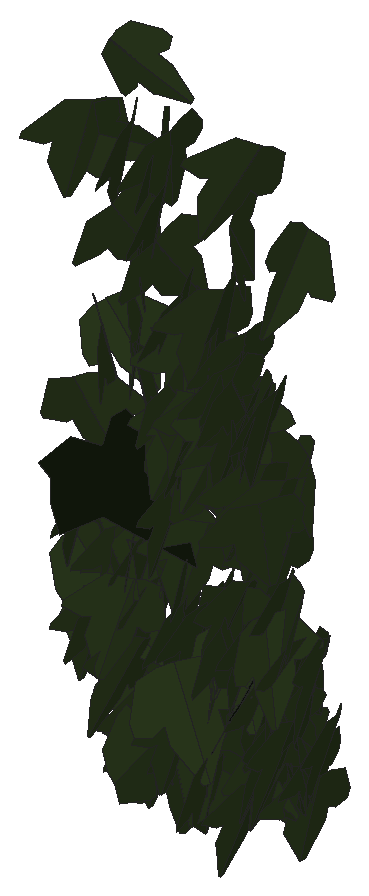
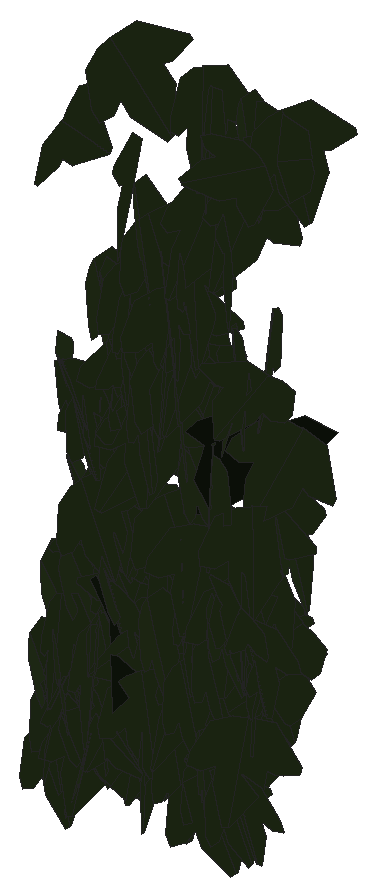
# SketchUp Ruby script. Lengths in inches.
U = 1.inch
M = Sketchup.active_model
def pt(a) = Geom::Point3d.new(a.map { |v| v * U })
def face(e, loops, mat)
  f = e.add_face(loops[0].map { |a| pt(a) })
  loops[1..].each { |l| e.add_face(l.map { |a| pt(a) }).erase! }
  f.material = f.back_material = mat if mat
  f
end
# faces: each face lists its corners as indices into pts; further lists are holes
def faces(e, pts, list, mat = nil) = list.each { |f| face(e, (f[0].is_a?(Array) ? f : [f]).map { |l| l.map { |i| pts[i] } }, mat) }
# xy, xz, yz: faces in a plane at the given z, y or x. An outline is a flat list of corners, or four numbers for a rectangle; further outlines are holes
def ring(l) = l.size == 4 ? [[l[0], l[1]], [l[2], l[1]], [l[2], l[3]], [l[0], l[3]]] : l.each_slice(2).to_a
def flat(e, list, mat, &to3) = list.each { |f| face(e, (f[0].is_a?(Array) ? f : [f]).map { |l| ring(l).map { |u, v| to3.(u, v) } }, mat) }
def xy(e, z, list, mat = nil) = flat(e, list, mat) { |x, y| [x, y, z] }
def xz(e, y, list, mat = nil) = flat(e, list, mat) { |x, z| [x, y, z] }
def yz(e, x, list, mat = nil) = flat(e, list, mat) { |y, z| [x, y, z] }
def lines(e, pts, list) = list.each { |a, b| e.add_line(pt(pts[a]), pt(pts[b])) }
# prism: a flat outline (further loops are holes) pulled along v
def prism(e, loops, v, mat = nil)
  f = face(e, loops, mat); d = Geom::Vector3d.new(v.map { |x| x * U })
  f.pushpull(f.normal.samedirection?(d) ? d.length : -d.length)
end
def box(e, o, s, mat = nil) = prism(e, [[o, [o[0] + s[0], o[1], o[2]], [o[0] + s[0], o[1] + s[1], o[2]], [o[0], o[1] + s[1], o[2]]]], [0, 0, s[2]], mat)
def at(x, y, z, deg = 0) = Geom::Transformation.translation(pt([x, y, z])) * Geom::Transformation.rotation(ORIGIN, Z_AXIS, deg.degrees)
def axes(o, x, y, z) = Geom::Transformation.new([*x, 0, *y, 0, *z, 0, *pt(o).to_a, 1])
def part(name) = M.definitions.add(name)
# library, detail: a bought-in or finely detailed component or shape, given as its bounding box
def library(name, o, s) = part(name).tap { |d| box(d.entities, o, s) }
def detail(e, o, s) = box(e.add_group.entities, o, s)
def put(e, d, t, mat = nil) = e.add_instance(d, t).tap { |i| i.material = mat if mat }
def group(e, t, mat = nil) = e.add_group.tap { |g| g.transformation = t; g.material = mat if mat }.entities
root = M.entities
M.materials.add("efeu1").color = [18, 25, 13]
M.materials.add("efeu2").color = [43, 57, 29]
c1 = part("ivyleaf_10")
p = [[0,0.5,-0.03],[-0.0625,2.02,-0.43],[-0.19,2.01,-0.46],[-0.54,1.05,-0.29],[-0.52,0.625,-0.18],[-0.83,0.76,-0.28],
  [-1.16,0.64,-0.33],[-1.15,0.33,-0.24],[-0.77,-0.39,0.02],[-0.3,-0.51,0.16],[0.04,-0.48,0.23],[-0.02,2.01,-0.4375],
  [-0.06,2.01,-0.43],[0.04,-0.49,0.23],[0.67,-0.49,0.14],[1.38,0.36,-0.2],[1.375,0.51,-0.24],[0.81,0.65,-0.19],
  [0.62,0.59,-0.15],[0.6,1.09,-0.28],[0.5,1.23,-0.31]]
faces(c1.entities,p,[[0,1,2,3,4,5,6,7,8,9,10],[11,12,0,13,14,15,16,17,18,19,20]],"efeu2")
c2 = part("ivyleaf_9")
p = [[1.54,2.16,1.25],[1.36,2.04,1.19],[-0.21,0.99,0.68],[-0.71,1.11,0.82],[-0.85,0.86,0.67],[-0.8,0.17,0.21],
  [-0.9,-0.01,0.1],[-0.67,-0.16,-0.02],[-0.08,-0.08,-0.05],[-0.03,-0.6,-0.4],[0.65,-0.88,-0.66],[0.83,-0.6,-0.49],
  [1.29,-0.42,-0.43],[1.8125,-0.07,-0.26],[1.21,0.44,0.15]]
faces(c2.entities,p,[[0,1,2,3,4,5,6,7,8,9,10,11,12,13,14]],"efeu1")
put(root,c1,axes([511.15,138.33,173.45],[-0.53133,-0.36546,-0.08051],[0.06901,0.04172,-0.64486],[0.3678,-0.53577,0.0047]))
put(root,c1,axes([511.1875,137.57,174.37],[-0.07517,-0.63344,0.13711],[0.02718,-0.14099,-0.63646],[0.64754,-0.06761,0.04263]))
put(root,c1,axes([511.03,137.4,177.95],[-0.62883,-0.1578,-0.2539],[0.25357,0.03165,-0.64769],[0.15833,-0.67742,0.02889]))
put(root,c1,axes([511.2,137.5,174.31],[-0.0367,-0.5542,-0.34902],[0.05334,0.34587,-0.55481],[0.65276,-0.05942,0.02571]))
put(root,c1,axes([511.25,137.1,176.54],[0.20511,-0.67223,-0.01479],[0.00018,0.01552,-0.70281],[0.6724,0.20506,0.0047]))
put(root,c1,axes([510.8,137.61,175.09],[0.46308,0.08973,0.46146],[0.45781,0.13491,-0.45439],[-0.1716,0.6021,0.03304]))
put(root,c1,axes([511.34,137.03,182.93],[-0.29651,-0.63131,0.13286],[-0.02442,-0.13513,-0.69661],[0.64468,-0.29549,0.03472]))
put(root,c1,axes([510.87,138.625,183.2],[-0.29498,-0.01649,-0.51058],[0.5277,-0.06697,-0.28036],[-0.05464,-0.5578,0.04875]))
put(root,c1,axes([510.94,138.64,175.75],[0.4809,-0.09085,0.34008],[0.34546,-0.06796,-0.47263],[0.12251,0.54826,-0.00224]))
put(root,c1,axes([511.21,138.05,175.04],[0.65936,-0.04096,-0.05098],[-0.04671,0.06659,-0.65758],[0.04577,0.65796,0.06338]))
put(root,c1,axes([511.38,137.85,176.66],[-0.52077,-0.41886,0.03252],[-0.00711,-0.043,-0.66769],[0.42006,-0.52001,0.02902]))
put(root,c1,axes([511.26,138.24,172.6],[0.65161,-0.20335,0.02645],[0.02522,-0.00797,-0.68261],[0.20351,0.6521,-0.0001]))
put(root,c1,axes([511.12,137.7,175.75],[-0.52464,0.14683,-0.37282],[0.31847,-0.23272,-0.5147],[-0.27132,-0.55707,0.11676]))
put(root,c1,axes([511.45,137.89,175.45],[-0.20993,-0.6397,-0.03572],[0.00516,0.0359,-0.67324],[0.64068,-0.2099,-0.00628]))
put(root,c1,axes([510.98,137.7,174.26],[0.33472,0.27444,0.5275],[0.38809,0.35781,-0.4324],[-0.45052,0.51212,0.01943]))
put(root,c1,axes([511.49,137.92,175.6],[0.35504,-0.46871,-0.31687],[-0.08504,0.32563,-0.57696],[0.55935,0.34702,0.11341]))
put(root,c1,axes([511.5,138.23,172.43],[-0.02758,-0.61533,0.16209],[0.03251,-0.16339,-0.61474],[0.63549,-0.01834,0.03848]))
put(root,c1,axes([511.57,137.98,175.37],[-0.3656,-0.54994,-0.10257],[0.08431,0.06697,-0.65956],[0.55304,-0.37376,0.03275]))
put(root,c1,axes([511.6,137.75,173.51],[0.00758,-0.57265,0.3385],[0.00865,-0.3384,-0.57269],[0.66516,0.01093,0.00359]))
put(root,c1,axes([511.25,137.83,179.11],[0.42155,0.29513,0.33107],[0.27307,0.19342,-0.50891],[-0.38109,0.46506,0.00156]))
put(root,c1,axes([511.7,138.06,175.33],[0.10458,-0.6555,0.0077],[-0.01596,-0.01034,-0.66356],[0.65535,0.10436,-0.01739]))
put(root,c1,axes([511.7,136.9,179.41],[0.38995,-0.4563,-0.37185],[-0.01203,0.43978,-0.55226],[0.58851,0.31134,0.23511]))
put(root,c1,axes([511.77,137.43,174.71],[-0.35506,-0.50671,0.22798],[0.00311,-0.27236,-0.60051],[0.55563,-0.32228,0.14905]))
put(root,c1,axes([511.26,137.13,182.5625],[0.17142,-0.08418,0.61824],[0.46785,0.44179,-0.05523],[-0.44896,0.42824,0.1785]))
put(root,c1,axes([511.9375,138.21,172.18],[-0.38663,-0.46937,0.22543],[-0.07868,-0.22489,-0.6032],[0.51472,-0.38694,0.07713]))
put(root,c1,axes([511.85,138.16,174.59],[0.04878,-0.6554,-0.01014],[-0.0002,0.01015,-0.65721],[0.65548,0.04877,0.00056]))
put(root,c1,axes([511.93,137.45,179.28],[0.41217,-0.49191,-0.26423],[-0.06963,0.28057,-0.63096],[0.55402,0.40123,0.11728]))
put(root,c1,axes([511.95,138.22,172.9],[0.20759,-0.57519,-0.19],[-0.04277,0.18643,-0.61111],[0.60425,0.2108,0.02202]))
put(root,c1,axes([512.01,137.625,172.52],[-0.0152,-0.64209,-0.11858],[0.01256,0.11831,-0.6422],[0.65283,-0.01723,0.00959]))
put(root,c1,axes([512.06,137.06,182.87],[0.23939,-0.66517,-0.10263],[-0.01169,0.10481,-0.70652],[0.67294,0.23844,0.02423]))
put(root,c1,axes([512.34,137.12,180.95],[-0.21157,0.41784,0.51326],[-0.42359,0.32854,-0.44207],[-0.50853,-0.44751,0.15469]))
put(root,c1,axes([512.04,136.95,181.56],[-0.26905,-0.54368,-0.37865],[0.17077,0.33796,-0.60661],[0.64015,-0.31866,0.00268]))
put(root,c1,axes([512.16,137.83,172.32],[-0.08214,-0.66371,0.02105],[-0.0003,-0.02118,-0.66877],[0.66405,-0.08211,0.00231]))
put(root,c1,axes([512.15,137.7,177.2],[0.49209,-0.44172,-0.14903],[0.05273,0.26804,-0.62036],[0.46319,0.43877,0.22895]))
put(root,c1,axes([512.02,137.51,178.69],[-0.36654,0.44971,-0.37639],[0.21445,-0.31033,-0.57963],[-0.54582,-0.42393,0.02503]))
put(root,c1,axes([512.28,137.85,176.02],[-0.59455,-0.29765,-0.08444],[0.09273,0.00307,-0.66378],[0.29517,-0.60051,0.03846]))
put(root,c1,axes([512.18,136.92,172.2],[0.0671,0.21097,-0.64366],[0.2053,0.61005,0.22136],[0.64549,-0.21596,-0.00349]))
put(root,c2,axes([511.98,136.68,177.61],[-0.05901,-0.38165,-0.68878],[0.1505,0.67252,-0.38553],[0.77293,-0.16009,0.02248]))
put(root,c1,axes([512.55,137.88,173.7],[-0.01342,-0.65638,0.0168],[-0.00529,-0.01669,-0.6565],[0.65658,-0.01355,-0.00495]))
put(root,c1,axes([512.67,137.08,182.85],[0.19003,-0.57376,-0.38438],[-0.05336,0.38528,-0.60148],[0.68855,0.18821,0.05947]))
put(root,c1,axes([512.7,137.92,172.49],[-0.02827,-0.65385,-0.01163],[-0.00667,0.01193,-0.65443],[0.65392,-0.02815,-0.00717]))
put(root,c1,axes([512.79,136.93,182.1],[0.19013,-0.65849,-0.24032],[-0.07022,0.22986,-0.68538],[0.69744,0.20265,-0.00349]))
put(root,c1,axes([512.79,137.64,175.64],[0.2884,-0.57359,-0.24048],[-0.02182,0.25558,-0.63578],[0.62158,0.27511,0.08925]))
put(root,c1,axes([512.81,137.41,174.77],[0.07086,-0.64045,-0.17021],[0.00638,0.17183,-0.6439],[0.66265,0.06683,0.0244]))
put(root,c1,axes([512.85,137.57,173.5],[-0.01933,-0.49141,-0.47177],[0.04592,0.46995,-0.49139],[0.67967,-0.04572,0.01978]))
put(root,c1,axes([512.93,137.1875,180.21],[0.0808,-0.66352,-0.23934],[-0.04887,0.23506,-0.66816],[0.70368,0.09251,-0.01892]))
put(root,c1,axes([512.82,137.01,181.1875],[-0.23526,-0.54082,-0.40317],[0.15837,0.37077,-0.58977],[0.65571,-0.28359,-0.00221]))
put(root,c1,axes([512.93,136.99,183.06],[-0.10108,-0.67884,-0.18934],[0.00661,0.19036,-0.68601],[0.70472,-0.09915,-0.02072]))
put(root,c1,axes([512.91,138.18,174.76],[0.13352,-0.64214,-0.01462],[-0.00702,0.01347,-0.65586],[0.64227,0.13364,-0.00412]))
put(root,c1,axes([512.95,137.34,173.11],[-0.0679,-0.63604,0.13574],[0.00556,-0.13704,-0.63935],[0.65034,-0.06524,0.01964]))
put(root,c1,axes([512.91,137.21,176.95],[0.13014,-0.63696,0.17304],[0.03828,-0.16879,-0.65011],[0.65894,0.13561,0.00359]))
put(root,c1,axes([513.19,137.14,171.78],[0.46474,-0.12951,0.46006],[-0.44306,0.12388,0.48245],[-0.17922,-0.6421,0.00029]))
put(root,c1,axes([512.99,137.03,178.82],[-0.1159,-0.54203,-0.39898],[0.11383,0.38324,-0.55371],[0.66335,-0.16047,0.02531]))
put(root,c1,axes([513.13,137.53,176.13],[-0.33046,-0.55119,0.19166],[-0.04559,-0.19519,-0.63997],[0.58177,-0.32838,0.05871]))
put(root,c1,axes([513.1,137.29,178.36],[-0.18619,-0.6015,0.31164],[0.00284,-0.32389,-0.62344],[0.67743,-0.16396,0.08827]))
put(root,c1,axes([513.21,137.36,179.48],[-0.51677,-0.47524,0.07532],[0.04077,-0.15338,-0.68803],[0.47944,-0.4992,0.13969]))
put(root,c1,axes([513.22,138.05,173.37],[-0.41186,-0.51185,0.09508],[0.02956,-0.14403,-0.64733],[0.51977,-0.3974,0.11216]))
put(root,c1,axes([513.24,137.4,174.94],[0.01032,-0.6808,-0.11343],[-0.01706,0.11316,-0.68071],[0.68997,0.01298,-0.01513]))
put(root,c1,axes([513.27,137.08,178.16],[0.24069,-0.62018,-0.23706],[-0.05204,0.23376,-0.66438],[0.6619,0.24389,0.03397]))
put(root,c1,axes([513.24,137.4375,179.93],[0.51893,-0.45673,-0.11867],[-0.00277,0.17343,-0.67962],[0.47189,0.50328,0.12651]))
put(root,c1,axes([513.29,137.3,178.72],[0.2338,-0.5929,-0.29713],[0.0359,0.32591,-0.62207],[0.66222,0.19166,0.13863]))
put(root,c1,axes([513.4,137.42,178.44],[-0.12113,-0.62782,0.29259],[-0.02907,-0.29216,-0.63893],[0.69204,-0.12216,0.02437]))
put(root,c1,axes([513.4375,137.6,177.77],[-0.58298,-0.36605,-0.00176],[-0.00323,0.00847,-0.68832],[0.36604,-0.58292,-0.00889]))
put(root,c1,axes([513.39,137.69,172.36],[0.17197,-0.5681,-0.25628],[0.00695,0.26759,-0.58851],[0.6232,0.15379,0.07728]))
put(root,c1,axes([513.21,137.05,178.18],[-0.47799,-0.28981,-0.39055],[0.35687,0.16301,-0.55773],[0.33039,-0.59534,0.03741]))
put(root,c1,axes([513.53,137.59,178.02],[0.08114,-0.66509,-0.15393],[-0.02152,0.15245,-0.67002],[0.68234,0.0839,-0.00283]))
put(root,c1,axes([513.68,137.95,171.97],[-0.24863,-0.32018,-0.50653],[-0.32199,-0.39112,0.40527],[-0.50538,0.40671,-0.00902]))
put(root,c1,axes([513.58,137.18,174.44],[0.42995,-0.46886,-0.18478],[-0.03177,0.21719,-0.62502],[0.50296,0.41453,0.11848]))
put(root,c1,axes([513.3,136.78,173.98],[0.58767,0.37901,0.26824],[0.21856,0.15596,-0.69919],[-0.40968,0.62689,0.01177]))
put(root,c1,axes([513.625,136.95,172.61],[0.19809,-0.62649,-0.21894],[0.01193,0.23181,-0.65252],[0.66354,0.18286,0.07709]))
put(root,c1,axes([513.69,137.18,180.45],[-0.20553,-0.66648,0.16178],[-0.01653,-0.16403,-0.69673],[0.68564,-0.20374,0.0317]))
put(root,c1,axes([513.48,137.4,177.46],[-0.3782,-0.44886,-0.43311],[0.29899,0.31407,-0.58657],[0.54742,-0.48164,0.02114]))
put(root,c1,axes([514.14,138.15,172.61],[-0.06744,0.12528,0.62325],[-0.63293,0.04537,-0.07761],[-0.05944,-0.62524,0.11925]))
put(root,c1,axes([513.71,137.34,178.35],[-0.10111,-0.51814,0.45118],[0.09384,-0.46218,-0.50974],[0.68061,-0.01325,0.1373]))
put(root,c1,axes([513.7,137.32,173.88],[-0.01572,-0.03598,-0.69138],[0.13889,0.67733,-0.03841],[0.67824,-0.13954,-0.00815]))
put(root,c1,axes([514.02,138.32,173.98],[-0.45545,0.33583,0.4292],[-0.35538,0.24103,-0.56572],[-0.41316,-0.57754,0.01348]))
put(root,c1,axes([513.81,137.36,178.13],[-0.11679,-0.67361,0.04651],[0.06611,-0.05838,-0.67954],[0.67197,-0.11133,0.07494]))
put(root,c1,axes([513.71,137.69,173.13],[-0.35736,-0.43856,-0.36402],[0.22763,0.28409,-0.56572],[0.52253,-0.42369,-0.00252]))
put(root,c1,axes([514,137.34,181.66],[-0.24059,0.46905,0.46053],[-0.32437,0.34183,-0.51761],[-0.57174,-0.39131,0.09987]))
put(root,c1,axes([513.73,137.54,178.49],[-0.53885,-0.3769,-0.19542],[0.22412,0.01565,-0.64817],[0.36057,-0.57297,0.11084]))
put(root,c1,axes([513.93,137.21,179.25],[-0.04867,-0.69172,0.02561],[-0.00156,-0.02556,-0.69343],[0.69219,-0.0487,0.00024]))
put(root,c1,axes([513.93,137.47,179.7],[-0.10647,-0.68909,-0.0452],[0.01171,0.04392,-0.69725],[0.69047,-0.107,0.00486]))
put(root,c1,axes([513.96,137.5,178.64],[-0.18765,0.64918,0.15496],[-0.19679,0.09999,-0.65722],[-0.63775,-0.22187,0.1572]))
put(root,c1,axes([513.89,137.42,179.32],[0.08353,-0.67056,-0.16265],[0.06531,0.17078,-0.67056],[0.68691,0.0653,0.08353]))
put(root,c1,axes([513.92,137.22,180.87],[0.28954,-0.64363,-0.11627],[-0.00346,0.12565,-0.70414],[0.65404,0.2856,0.04775]))
put(root,c1,axes([513.75,138.01,174.84],[0.61112,-0.26994,0.16014],[0.14102,-0.07699,-0.66795],[0.2804,0.62704,-0.01308]))
put(root,c2,axes([514.21,136.95,173.8],[-0.04453,0.53285,0.54734],[-0.02689,0.54684,-0.53455],[-0.76341,-0.05034,-0.0131]))
put(root,c1,axes([514.01,137.63,175.1],[0.10254,-0.60463,0.26286],[0.02786,-0.26181,-0.61308],[0.65871,0.1052,-0.01499]))
put(root,c1,axes([513.57,137.88,172.35],[-0.23337,0.07954,-0.60477],[0.56036,-0.22786,-0.2462],[-0.24099,-0.60687,0.01317]))
put(root,c1,axes([513.78,137.48,174.57],[0.58208,0.24251,0.22579],[0.20542,0.09401,-0.63054],[-0.25999,0.61722,0.00732]))
put(root,c1,axes([514.04,136.875,175.04],[0.06914,-0.58898,-0.31305],[0.06596,0.31922,-0.58602],[0.66373,0.02963,0.09085]))
put(root,c1,axes([514.09,137.3,178.73],[0.07889,-0.68053,0.16412],[0.01819,-0.16311,-0.68509],[0.69981,0.08096,-0.0007]))
put(root,c1,axes([514.09,137.17,175.59],[0.09688,-0.61001,0.28124],[0.03127,-0.27975,-0.61754],[0.67099,0.10112,-0.01182]))
put(root,c1,axes([513.99,137.3,175.43],[-0.66468,-0.01113,-0.20775],[0.20748,0.01547,-0.66468],[0.01523,-0.69622,-0.01144]))
put(root,c1,axes([514.17,137.39,172.14],[0.01291,-0.63852,0.17564],[-0.01395,-0.1759,-0.63843],[0.66209,0.00874,-0.01688]))
put(root,c1,axes([514.34,137.12,183.17],[-0.24732,-0.58792,0.33025],[-0.13506,-0.30145,-0.63779],[0.66066,-0.28171,-0.00675]))
put(root,c1,axes([514.24,138.04,176.23],[-0.17408,-0.62171,0.15575],[-0.01522,-0.15734,-0.64506],[0.64074,-0.17265,0.027]))
put(root,c1,axes([514.21,137.7,173.85],[0.07826,-0.65679,0.00898],[0.00075,-0.00896,-0.66144],[0.65685,0.07827,-0.00032]))
put(root,c1,axes([514.15,138.08,172.47],[-0.39353,-0.50942,-0.15101],[0.14593,0.07706,-0.64027],[0.5109,-0.4144,0.06657]))
put(root,c1,axes([514.23,136.92,179.34],[-0.02803,-0.5891,-0.3551],[0.04879,0.3528,-0.58913],[0.68612,-0.04915,0.02738]))
put(root,c1,axes([514.24,138.2,172.34],[-0.44063,0.45851,0.01765],[-0.02414,0.00127,-0.6357],[-0.45821,-0.44098,0.01652]))
put(root,c1,axes([514.27,137.36,175.03],[0.15373,-0.66291,0.10212],[0.0198,-0.10024,-0.6805],[0.67044,0.15496,-0.00332]))
put(root,c1,axes([514.4,137.26,177.6875],[-0.14152,-0.64937,0.18779],[-0.03324,-0.18494,-0.66458],[0.67516,-0.14522,0.00664]))
put(root,c1,axes([514.39,138.05,172.75],[0.00327,-0.49757,0.40547],[0.07626,-0.4023,-0.4943],[0.63731,0.05069,0.05707]))
put(root,c1,axes([514.47,137.52,173.22],[0.22291,-0.54803,0.2909],[0.0933,-0.27598,-0.59141],[0.61339,0.24113,-0.01575]))
put(root,c1,axes([514.58,137.72,173.49],[-0.15317,-0.57233,-0.33623],[0.09045,0.32385,-0.59247],[0.6576,-0.17786,0.00318]))
put(root,c1,axes([514.64,138.15,172.9],[-0.26432,0.52876,0.26016],[-0.1574,0.21143,-0.58963],[-0.56789,-0.30471,0.04234]))
put(root,c1,axes([514.65,137.37,177.43],[-0.12807,-0.65332,0.20822],[0.0012,-0.21203,-0.66455],[0.68569,-0.12165,0.04006]))
put(root,c1,axes([514.6,138.23,174.25],[0.07417,-0.5951,-0.25983],[0.03758,0.26502,-0.59624],[0.64826,0.05273,0.0643]))
put(root,c1,axes([514.59,137.12,179.18],[0.36217,-0.57965,0.04082],[0.01568,-0.03833,-0.68345],[0.58087,0.36244,-0.00699]))
put(root,c1,axes([514.7,138.1,173.76],[0.21599,-0.59554,-0.18444],[-0.03531,0.1832,-0.63287],[0.62244,0.21704,0.0281]))
put(root,c1,axes([514.81,137.6875,177.86],[0.55259,-0.26567,-0.34608],[-0.24116,0.2794,-0.59957],[0.36358,0.58912,0.12829]))
put(root,c1,axes([514.75,138.21,172.13],[-0.18343,-0.62597,0.04653],[-0.01848,-0.04307,-0.65227],[0.62742,-0.18427,-0.00561]))
put(root,c1,axes([514.65,137.58,173.21],[0.1752,-0.61482,0.26618],[0.07238,-0.25615,-0.6393],[0.66605,0.18956,-0.00055]))
put(root,c1,axes([514.74,136.93,177.34],[-0.41908,-0.54577,-0.09012],[0.04401,0.07981,-0.68797],[0.55141,-0.42116,-0.01359]))
put(root,c1,axes([514.71,137.4375,175.76],[0.2623,-0.63727,0.14417],[0.04448,-0.13757,-0.68905],[0.65186,0.26582,-0.01099]))
put(root,c1,axes([514.83,138.22,172.72],[0.05328,-0.6501,-0.05822],[-0.00788,0.05777,-0.65228],[0.65266,0.05377,-0.00312]))
put(root,c1,axes([514.83,136.99,179.2],[0.15182,-0.69872,-0.00348],[0.00233,0.00407,-0.71502],[0.69872,0.15181,0.00314]))
put(root,c1,axes([514.94,137.47,174.79],[0.1662,-0.64425,0.18527],[0.04396,-0.17999,-0.66534],[0.66891,0.1719,-0.00231]))
put(root,c1,axes([514.88,136.93,175.3],[0.14303,0.66193,-0.02644],[-0.00575,-0.02581,-0.67721],[-0.66243,0.14314,0.00017]))
put(root,c1,axes([514.96,137.67,178.01],[0.47299,-0.49863,0.15825],[0.11029,-0.11351,-0.68728],[0.51139,0.48568,0.00185]))
put(root,c1,axes([515.0625,137.89,174.63],[0.23615,-0.53655,0.27118],[0.131,-0.23842,-0.58582],[0.58674,0.26918,0.02165]))
put(root,c1,axes([515.17,138.02,173.37],[0.23974,-0.59477,0.09252],[0.02487,-0.08971,-0.64118],[0.60141,0.2408,-0.01037]))
put(root,c1,axes([515.23,137.09,175.87],[0.4443,-0.50245,-0.0583],[-0.03592,0.04605,-0.6707],[0.50454,0.44573,0.00358]))
put(root,c1,axes([515.21,137.3125,181.86],[0.09889,0.49572,-0.49573],[-0.09618,-0.48631,-0.50549],[-0.69443,0.13795,-0.00058]))
